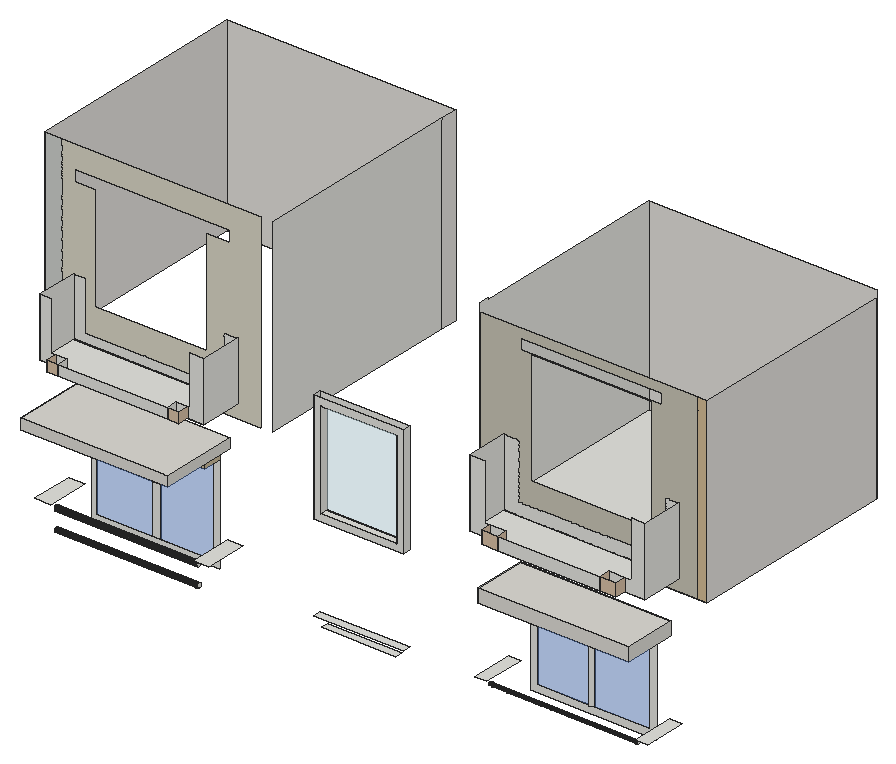
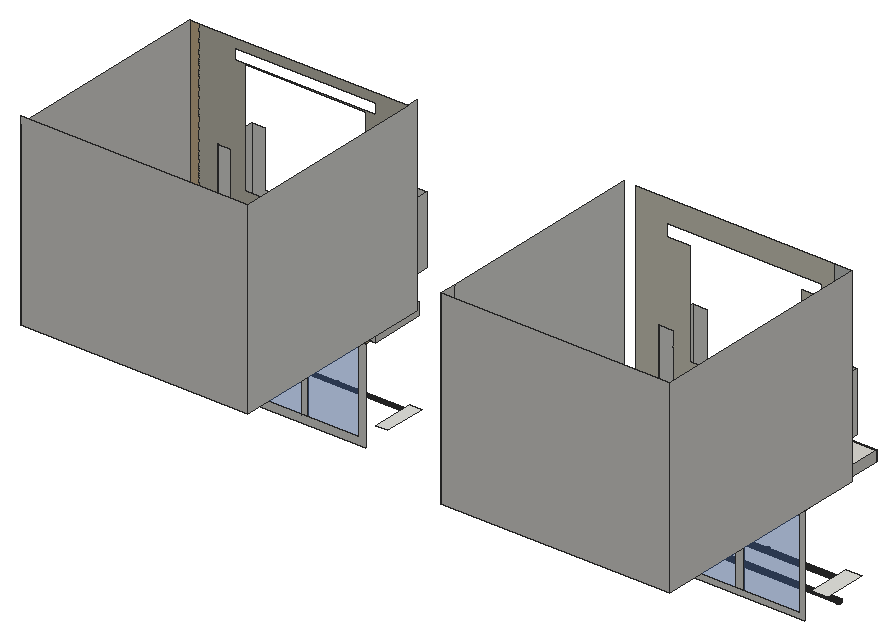
# SketchUp Ruby script. Lengths in inches.
U = 1.inch
M = Sketchup.active_model
def pt(a) = Geom::Point3d.new(a.map { |v| v * U })
def face(e, loops, mat)
  f = e.add_face(loops[0].map { |a| pt(a) })
  loops[1..].each { |l| e.add_face(l.map { |a| pt(a) }).erase! }
  f.material = f.back_material = mat if mat
  f
end
# faces: each face lists its corners as indices into pts; further lists are holes
def faces(e, pts, list, mat = nil) = list.each { |f| face(e, (f[0].is_a?(Array) ? f : [f]).map { |l| l.map { |i| pts[i] } }, mat) }
# xy, xz, yz: faces in a plane at the given z, y or x. An outline is a flat list of corners, or four numbers for a rectangle; further outlines are holes
def ring(l) = l.size == 4 ? [[l[0], l[1]], [l[2], l[1]], [l[2], l[3]], [l[0], l[3]]] : l.each_slice(2).to_a
def flat(e, list, mat, &to3) = list.each { |f| face(e, (f[0].is_a?(Array) ? f : [f]).map { |l| ring(l).map { |u, v| to3.(u, v) } }, mat) }
def xy(e, z, list, mat = nil) = flat(e, list, mat) { |x, y| [x, y, z] }
def xz(e, y, list, mat = nil) = flat(e, list, mat) { |x, z| [x, y, z] }
def yz(e, x, list, mat = nil) = flat(e, list, mat) { |y, z| [x, y, z] }
def lines(e, pts, list) = list.each { |a, b| e.add_line(pt(pts[a]), pt(pts[b])) }
# prism: a flat outline (further loops are holes) pulled along v
def prism(e, loops, v, mat = nil)
  f = face(e, loops, mat); d = Geom::Vector3d.new(v.map { |x| x * U })
  f.pushpull(f.normal.samedirection?(d) ? d.length : -d.length)
end
def box(e, o, s, mat = nil) = prism(e, [[o, [o[0] + s[0], o[1], o[2]], [o[0] + s[0], o[1] + s[1], o[2]], [o[0], o[1] + s[1], o[2]]]], [0, 0, s[2]], mat)
def at(x, y, z, deg = 0) = Geom::Transformation.translation(pt([x, y, z])) * Geom::Transformation.rotation(ORIGIN, Z_AXIS, deg.degrees)
def axes(o, x, y, z) = Geom::Transformation.new([*x, 0, *y, 0, *z, 0, *pt(o).to_a, 1])
def part(name) = M.definitions.add(name)
# library, detail: a bought-in or finely detailed component or shape, given as its bounding box
def library(name, o, s) = part(name).tap { |d| box(d.entities, o, s) }
def detail(e, o, s) = box(e.add_group.entities, o, s)
def put(e, d, t, mat = nil) = e.add_instance(d, t).tap { |i| i.material = mat if mat }
def group(e, t, mat = nil) = e.add_group.tap { |g| g.transformation = t; g.material = mat if mat }.entities
root = M.entities
M.materials.add("[Basic Tile]").color = [203, 206, 202]
M.materials.add("[Color M07]").color = [58, 58, 58]
M.materials.add("[Formica Beige]").color = [211, 187, 149]
M.materials.add("[Formica Graystone]").color = [198, 194, 180]
M.materials.add("[Formica Graystone]1").color = [216, 212, 196]
M.materials.add("[Formica Laminate Dark]").color = [50, 53, 60]
M.materials.add("[Formica Laminate Light]").color = [213, 189, 164]
M.materials.add("[Quartz Light Brown]").color = [199, 184, 152]
M.materials.add("[Terrazzo Tile Accent]").color = [224, 221, 217]
M.materials.add("[Terrazzo Tile Light]").color = [219, 217, 210]
M.materials.add("[Translucent Glass Blue]").color = [85, 126, 201]
M.materials["[Translucent Glass Blue]"].alpha = 0.5
M.materials.add("[Translucent Glass Safety]").color = [204, 235, 244]
M.materials["[Translucent Glass Safety]"].alpha = 0.5
xy(root,378.64,[[183.77,109.54,226.43,114.1]])
xy(root,383,[[179.41,109.54,230.79,114.1]])
xy(root,395.85,[[296.64,90.87,296.85,90.9,297.04,90.98,297.21,91.11,297.34,91.28,297.42,91.47,297.45,91.68,297.42,91.89,297.34,92.09,297.21,92.26,297.04,92.39,296.85,92.47,296.64,92.5,296.43,92.47,296.23,92.39,296.0625,92.26,295.93,92.09,295.85,91.89,295.82,91.68,295.85,91.47,295.93,91.28,296.0625,91.11,296.23,90.98,296.43,90.9]],"[Formica Laminate Dark]")
xy(root,395.97,[[324.82,90.87,325.03,90.9,325.23,90.98,325.4,91.11,325.53,91.28,325.61,91.47,325.64,91.68,325.61,91.89,325.53,92.09,325.4,92.26,325.23,92.39,325.03,92.47,324.82,92.5,324.61,92.47,324.42,92.39,324.25,92.26,324.12,92.09,324.04,91.89,324.01,91.68,324.04,91.47,324.12,91.28,324.25,91.11,324.42,90.98,324.61,90.9]],"[Formica Laminate Dark]")
xy(root,396.04,[[305.39,90.87,305.6,90.9,305.79,90.98,305.96,91.11,306.09,91.28,306.17,91.47,306.2,91.68,306.17,91.89,306.09,92.09,305.96,92.26,305.79,92.39,305.6,92.47,305.39,92.5,305.18,92.47,304.98,92.39,304.8125,92.26,304.68,92.09,304.6,91.89,304.57,91.68,304.6,91.47,304.68,91.28,304.8125,91.11,304.98,90.98,305.18,90.9],[330.07,90.87,330.28,90.9,330.48,90.98,330.65,91.11,330.78,91.28,330.86,91.47,330.89,91.68,330.86,91.89,330.78,92.09,330.65,92.26,330.48,92.39,330.28,92.47,330.07,92.5,329.86,92.47,329.67,92.39,329.5,92.26,329.37,92.09,329.29,91.89,329.26,91.68,329.29,91.47,329.37,91.28,329.5,91.11,329.67,90.98,329.86,90.9]],"[Formica Laminate Dark]")
xy(root,396.16,[[310.2,90.87,310.41,90.9,310.6,90.98,310.77,91.11,310.9,91.28,310.98,91.47,311.01,91.68,310.98,91.89,310.9,92.09,310.77,92.26,310.6,92.39,310.41,92.47,310.2,92.5,309.99,92.47,309.79,92.39,309.625,92.26,309.49,92.09,309.41,91.89,309.39,91.68,309.41,91.47,309.49,91.28,309.625,91.11,309.79,90.98,309.99,90.9],[340.51,90.87,340.72,90.9,340.92,90.98,341.09,91.11,341.21,91.28,341.3,91.47,341.32,91.68,341.3,91.89,341.21,92.09,341.09,92.26,340.92,92.39,340.72,92.47,340.51,92.5,340.3,92.47,340.1,92.39,339.9375,92.26,339.81,92.09,339.73,91.89,339.7,91.68,339.73,91.47,339.81,91.28,339.9375,91.11,340.1,90.98,340.3,90.9],[345.89,90.87,346.1,90.9,346.29,90.98,346.46,91.11,346.59,91.28,346.67,91.47,346.7,91.68,346.67,91.89,346.59,92.09,346.46,92.26,346.29,92.39,346.1,92.47,345.89,92.5,345.68,92.47,345.48,92.39,345.3125,92.26,345.18,92.09,345.1,91.89,345.07,91.68,345.1,91.47,345.18,91.28,345.3125,91.11,345.48,90.98,345.68,90.9]],"[Formica Laminate Dark]")
xy(root,396.29,[[319.89,90.87,320.1,90.9,320.29,90.98,320.46,91.11,320.59,91.28,320.67,91.47,320.7,91.68,320.67,91.89,320.59,92.09,320.46,92.26,320.29,92.39,320.1,92.47,319.89,92.5,319.68,92.47,319.48,92.39,319.3125,92.26,319.18,92.09,319.1,91.89,319.07,91.68,319.1,91.47,319.18,91.28,319.3125,91.11,319.48,90.98,319.68,90.9],[356.89,90.87,357.1,90.9,357.29,90.98,357.46,91.11,357.59,91.28,357.67,91.47,357.7,91.68,357.67,91.89,357.59,92.09,357.46,92.26,357.29,92.39,357.1,92.47,356.89,92.5,356.68,92.47,356.48,92.39,356.3125,92.26,356.18,92.09,356.1,91.89,356.07,91.68,356.1,91.47,356.18,91.28,356.3125,91.11,356.48,90.98,356.68,90.9],[369.07,90.87,369.28,90.9,369.48,90.98,369.65,91.11,369.78,91.28,369.86,91.47,369.89,91.68,369.86,91.89,369.78,92.09,369.65,92.26,369.48,92.39,369.28,92.47,369.07,92.5,368.86,92.47,368.67,92.39,368.5,92.26,368.37,92.09,368.29,91.89,368.26,91.68,368.29,91.47,368.37,91.28,368.5,91.11,368.67,90.98,368.86,90.9]],"[Formica Laminate Dark]")
xy(root,396.35,[[314.77,91,315.63,91,315.77,91.11,315.9,91.28,315.98,91.47,316.01,91.68,315.98,91.89,315.9,92.09,315.77,92.26,315.6,92.39,315.41,92.47,315.2,92.5,314.99,92.47,314.79,92.39,314.625,92.26,314.49,92.09,314.41,91.89,314.39,91.68,314.41,91.47,314.49,91.28,314.625,91.11]])
xy(root,396.35,[[315.2,90.87,315.41,90.9,315.6,90.98,315.63,91,314.77,91,314.79,90.98,314.99,90.9],[351.2,90.87,351.41,90.9,351.6,90.98,351.77,91.11,351.9,91.28,351.98,91.47,352.01,91.68,351.98,91.89,351.9,92.09,351.77,92.26,351.6,92.39,351.41,92.47,351.2,92.5,350.99,92.47,350.79,92.39,350.625,92.26,350.49,92.09,350.41,91.89,350.39,91.68,350.41,91.47,350.49,91.28,350.625,91.11,350.79,90.98,350.99,90.9]],"[Formica Laminate Dark]")
xy(root,396.41,[[374.64,90.87,374.85,90.9,375.04,90.98,375.21,91.11,375.34,91.28,375.42,91.47,375.45,91.68,375.42,91.89,375.34,92.09,375.21,92.26,375.04,92.39,374.85,92.47,374.64,92.5,374.43,92.47,374.23,92.39,374.0625,92.26,373.93,92.09,373.85,91.89,373.82,91.68,373.85,91.47,373.93,91.28,374.0625,91.11,374.23,90.98,374.43,90.9]],"[Formica Laminate Dark]")
xy(root,396.54,[[363.01,90.87,363.22,90.9,363.42,90.98,363.59,91.11,363.71,91.28,363.8,91.47,363.82,91.68,363.8,91.89,363.71,92.09,363.59,92.26,363.42,92.39,363.22,92.47,363.01,92.5,362.8,92.47,362.6,92.39,362.4375,92.26,362.31,92.09,362.23,91.89,362.2,91.68,362.23,91.47,362.31,91.28,362.4375,91.11,362.6,90.98,362.8,90.9]],"[Formica Laminate Dark]")
xy(root,396.5625,[[300.61,91.03,301.54,91.03,301.65,91.11,301.78,91.28,301.86,91.47,301.89,91.68,301.86,91.89,301.78,92.09,301.65,92.26,301.48,92.39,301.28,92.47,301.07,92.5,300.86,92.47,300.67,92.39,300.5,92.26,300.37,92.09,300.29,91.89,300.26,91.68,300.29,91.47,300.37,91.28,300.5,91.11],[334.45,91.03,336.43,91.03,336.47,91.08,336.59,91.37,336.63,91.67,336.59,91.98,336.47,92.27,336.28,92.51,336.17,92.6,334.71,92.6,334.6,92.51,334.41,92.27,334.29,91.98,334.25,91.67,334.29,91.37,334.41,91.08]])
xy(root,396.5625,[[335.44,90.49,335.75,90.53,336.03,90.64,336.28,90.83,336.43,91.03,334.45,91.03,334.6,90.83,334.85,90.64,335.13,90.53],[301.07,90.87,301.28,90.9,301.48,90.98,301.54,91.03,300.61,91.03,300.67,90.98,300.86,90.9],[334.71,92.6,336.17,92.6,336.03,92.7,335.75,92.82,335.44,92.86,335.13,92.82,334.85,92.7]],"[Formica Laminate Dark]")
xy(root,397.9,[[52.52,92.0625,52.78,92.1,53.02,92.2,53.23,92.35,53.39,92.5625,53.49,92.8,53.52,93.0625,53.49,93.32,53.39,93.5625,53.23,93.77,53.02,93.93,52.78,94.03,52.52,94.0625,52.27,94.03,52.02,93.93,51.82,93.77,51.66,93.5625,51.56,93.32,51.52,93.0625,51.56,92.8,51.66,92.5625,51.82,92.35,52.02,92.2,52.27,92.1]])
xy(root,397.9,[[63.21,92.0625,63.47,92.1,63.71,92.2,63.92,92.35,64.08,92.5625,64.18,92.8,64.21,93.0625,64.18,93.32,64.08,93.5625,63.92,93.77,63.71,93.93,63.47,94.03,63.21,94.0625,62.95,94.03,62.71,93.93,62.5,93.77,62.35,93.5625,62.25,93.32,62.21,93.0625,62.25,92.8,62.35,92.5625,62.5,92.35,62.71,92.2,62.95,92.1]],"[Color M07]")
xy(root,398.08,[[47.34,92.0625,47.6,92.1,47.84,92.2,48.04,92.35,48.2,92.5625,48.3,92.8,48.34,93.0625,48.3,93.32,48.2,93.5625,48.04,93.77,47.84,93.93,47.6,94.03,47.34,94.0625,47.08,94.03,46.84,93.93,46.63,93.77,46.47,93.5625,46.37,93.32,46.34,93.0625,46.37,92.8,46.47,92.5625,46.63,92.35,46.84,92.2,47.08,92.1]])
xy(root,398.08,[[81.59,92.0625,81.85,92.1,82.09,92.2,82.29,92.35,82.45,92.5625,82.55,92.8,82.59,93.0625,82.55,93.32,82.45,93.5625,82.29,93.77,82.09,93.93,81.85,94.03,81.59,94.0625,81.33,94.03,81.09,93.93,80.88,93.77,80.72,93.5625,80.62,93.32,80.59,93.0625,80.62,92.8,80.72,92.5625,80.88,92.35,81.09,92.2,81.33,92.1]],"[Color M07]")
xy(root,398.15,[[56.96,92.0625,57.22,92.1,57.46,92.2,57.67,92.35,57.83,92.5625,57.93,92.8,57.96,93.0625,57.93,93.32,57.83,93.5625,57.67,93.77,57.46,93.93,57.22,94.03,56.96,94.0625,56.7,94.03,56.46,93.93,56.25,93.77,56.1,93.5625,56,93.32,55.96,93.0625,56,92.8,56.1,92.5625,56.25,92.35,56.46,92.2,56.7,92.1]])
xy(root,398.15,[[69.96,92.0625,70.22,92.1,70.46,92.2,70.67,92.35,70.83,92.5625,70.93,92.8,70.96,93.0625,70.93,93.32,70.83,93.5625,70.67,93.77,70.46,93.93,70.22,94.03,69.96,94.0625,69.7,94.03,69.46,93.93,69.25,93.77,69.1,93.5625,69,93.32,68.96,93.0625,69,92.8,69.1,92.5625,69.25,92.35,69.46,92.2,69.7,92.1],[76.09,92.0625,76.35,92.1,76.59,92.2,76.79,92.35,76.95,92.5625,77.05,92.8,77.09,93.0625,77.05,93.32,76.95,93.5625,76.79,93.77,76.59,93.93,76.35,94.03,76.09,94.0625,75.83,94.03,75.59,93.93,75.38,93.77,75.22,93.5625,75.12,93.32,75.09,93.0625,75.12,92.8,75.22,92.5625,75.38,92.35,75.59,92.2,75.83,92.1],[94.65,92.0625,94.91,92.1,95.15,92.2,95.36,92.35,95.52,92.5625,95.62,92.8,95.65,93.0625,95.62,93.32,95.52,93.5625,95.36,93.77,95.15,93.93,94.91,94.03,94.65,94.0625,94.39,94.03,94.15,93.93,93.94,93.77,93.78,93.5625,93.68,93.32,93.65,93.0625,93.68,92.8,93.78,92.5625,93.94,92.35,94.15,92.2,94.39,92.1]],"[Color M07]")
xy(root,398.4,[[122.21,92.0625,122.47,92.1,122.71,92.2,122.92,92.35,123.08,92.5625,123.18,92.8,123.21,93.0625,123.18,93.32,123.08,93.5625,122.92,93.77,122.71,93.93,122.47,94.03,122.21,94.0625,121.95,94.03,121.71,93.93,121.5,93.77,121.35,93.5625,121.25,93.32,121.21,93.0625,121.25,92.8,121.35,92.5625,121.5,92.35,121.71,92.2,121.95,92.1]],"[Color M07]")
xy(root,398.46,[[100.02,92.0625,100.28,92.1,100.52,92.2,100.73,92.35,100.89,92.5625,100.99,92.8,101.02,93.0625,100.99,93.32,100.89,93.5625,100.73,93.77,100.52,93.93,100.28,94.03,100.02,94.0625,99.77,94.03,99.52,93.93,99.32,93.77,99.16,93.5625,99.06,93.32,99.02,93.0625,99.06,92.8,99.16,92.5625,99.32,92.35,99.52,92.2,99.77,92.1]],"[Color M07]")
xy(root,398.47,[[287.58,89.73,294.32,114.1],[379.76,89.73,386.54,114.1]])
xy(root,398.52,[[105.1,92.28,106.32,92.28,106.42,92.35,106.58,92.5625,106.68,92.8,106.71,93.0625,106.68,93.32,106.58,93.5625,106.42,93.77,106.21,93.93,105.97,94.03,105.71,94.0625,105.45,94.03,105.21,93.93,105,93.77,104.85,93.5625,104.75,93.32,104.71,93.0625,104.75,92.8,104.85,92.5625,105,92.35],[111.17,92.28,112.38,92.28,112.48,92.35,112.64,92.5625,112.74,92.8,112.77,93.0625,112.74,93.32,112.64,93.5625,112.48,93.77,112.27,93.93,112.03,94.03,111.77,94.0625,111.52,94.03,111.27,93.93,111.07,93.77,110.91,93.5625,110.81,93.32,110.77,93.0625,110.81,92.8,110.91,92.5625,111.07,92.35]])
xy(root,398.52,[[105.71,92.0625,105.97,92.1,106.21,92.2,106.32,92.28,105.1,92.28,105.21,92.2,105.45,92.1],[111.77,92.0625,112.03,92.1,112.27,92.2,112.38,92.28,111.17,92.28,111.27,92.2,111.52,92.1]],"[Color M07]")
xy(root,398.65,[[117.4,92.0625,117.66,92.1,117.9,92.2,118.11,92.35,118.27,92.5625,118.37,92.8,118.4,93.0625,118.37,93.32,118.27,93.5625,118.11,93.77,117.9,93.93,117.66,94.03,117.4,94.0625,117.14,94.03,116.9,93.93,116.69,93.77,116.53,93.5625,116.43,93.32,116.4,93.0625,116.43,92.8,116.53,92.5625,116.69,92.35,116.9,92.2,117.14,92.1]],"[Color M07]")
xy(root,398.83,[[86.3,92.4,89.26,92.4,89.35,92.62,89.41,93.04,89.35,93.46,89.1875,93.85,88.93,94.19,88.59,94.45,88.31,94.57,87.26,94.57,86.97,94.45,86.63,94.19,86.375,93.85,86.21,93.46,86.16,93.04,86.21,92.62],[87.26,94.57,88.31,94.57,88.2,94.61,87.78,94.67,87.36,94.61]])
xy(root,398.83,[[87.78,91.42,88.2,91.47,88.59,91.63,88.93,91.89,89.1875,92.23,89.26,92.4,86.3,92.4,86.375,92.23,86.63,91.89,86.97,91.63,87.36,91.47]],"[Color M07]")
xy(root,401.52,[[35.74,89.73,44.74,114.1],[126.56,89.73,135.17,114.1]])
xy(root,432.625,[[179.41,109.54,230.79,114.1]])
xy(root,436.61,[[183.4,109.54,226.8,114.1]])
xy(root,438.74,[[299.92,104.54,372.17,114.1]],"[Quartz Light Brown]")
xy(root,439.98,[[299.92,104.54,372.17,105.1],[299.92,105.1,372.17,114.1]])
xy(root,440.81,[[48.8,103.54,121.8,114.1]],"[Quartz Light Brown]")
xy(root,441.22,[[299.92,105.1,372.17,114.1]])
xy(root,441.22,[[[294.2,83.54,294.2,114.1,299.92,114.1,299.92,105.1,372.17,105.1,372.17,114.1,380.45,114.1,380.45,83.54],[373.86,85.05,374.25,85.1,374.61,85.25,374.92,85.49,375.16,85.8,375.3125,86.17,375.36,86.55,375.3125,86.94,375.16,87.3,374.92,87.61,374.61,87.85,374.25,88,373.86,88.05,373.47,88,373.11,87.85,372.8,87.61,372.5625,87.3,372.41,86.94,372.36,86.55,372.41,86.17,372.5625,85.8,372.8,85.49,373.11,85.25,373.47,85.1],[299.55,85.05,299.9375,85.1,300.3,85.25,300.61,85.49,300.85,85.8,301,86.17,301.05,86.55,301,86.94,300.85,87.3,300.61,87.61,300.3,87.85,299.9375,88,299.55,88.05,299.16,88,298.8,87.85,298.49,87.61,298.25,87.3,298.1,86.94,298.05,86.55,298.1,86.17,298.25,85.8,298.49,85.49,298.8,85.25,299.16,85.1]]],"[Terrazzo Tile Light]")
xy(root,444.62,[[48.8,103.54,121.8,107.85],[48.8,107.85,121.8,114.1]])
xy(root,448.43,[[48.8,107.85,121.8,114.1]])
xy(root,448.43,[[43.4,69.48,48.8,114.1],[[48.8,69.48,121.8,107.85],[119,85,119.42,85.06,119.8125,85.22,120.15,85.48,120.41,85.82,120.57,86.21,120.625,86.63,120.57,87.05,120.41,87.44,120.15,87.78,119.8125,88.04,119.42,88.2,119,88.25,118.58,88.2,118.1875,88.04,117.85,87.78,117.59,87.44,117.43,87.05,117.375,86.63,117.43,86.21,117.59,85.82,117.85,85.48,118.1875,85.22,118.58,85.06],[51.5,85,51.92,85.06,52.3125,85.22,52.65,85.48,52.91,85.82,53.07,86.21,53.125,86.63,53.07,87.05,52.91,87.44,52.65,87.78,52.3125,88.04,51.92,88.2,51.5,88.25,51.08,88.2,50.6875,88.04,50.35,87.78,50.09,87.44,49.93,87.05,49.875,86.63,49.93,86.21,50.09,85.82,50.35,85.48,50.6875,85.22,51.08,85.06]],[121.8,69.48,127.71,114.1]],"[Terrazzo Tile Light]")
xy(root,448.85,[[294.2,83.54,380.45,114.1]],"[Terrazzo Tile Light]")
xy(root,454.37,[[43.4,69.48,127.71,114.1]],"[Terrazzo Tile Light]")
xy(root,465.6875,[[270.97,114.1,401.16,235.11]])
xy(root,472.29,[[305.49,83.42,305.49,89.73,284.68,89.73,284.68,114.1,384.86,114.1,384.86,89.73,364.3,89.73,364.3,83.42]])
xy(root,472.29,[[296.37,83.42,305.49,89.73],[364.3,83.42,373.43,89.73]],"[Formica Laminate Light]")
xy(root,473.3,[[53.75,83.48,53.75,89.73,38.09,89.73,38.09,114.1,132.15,114.1,132.15,89.73,116.48,89.73,116.48,83.48]])
xy(root,473.3,[[47.29,83.48,53.75,89.73],[116.48,83.48,122.94,89.73]],"[Formica Laminate Light]")
xz(root,69.48,[[43.4,448.43,127.71,454.37]],"[Terrazzo Tile Light]")
xz(root,83.42,[[305.49,472.29,364.3,479.47]])
xz(root,83.42,[[296.37,472.29,305.49,479.47],[364.3,472.29,373.43,479.47]],"[Formica Laminate Light]")
xz(root,83.48,[[53.75,473.3,116.48,479.18]])
xz(root,83.48,[[47.29,473.3,53.75,479.18],[116.48,473.3,122.94,479.18]],"[Formica Laminate Light]")
xz(root,83.54,[[294.2,441.22,380.45,448.85]],"[Terrazzo Tile Light]")
xz(root,89.73,[[284.68,472.29,296.37,472.29,296.37,479.47,293.32,479.47,293.32,511.22,284.68,511.22],[296.37,472.29,305.49,479.47],[364.3,472.29,373.43,479.47],[373.43,472.29,384.86,472.29,384.86,511.22,377.32,511.22,377.32,479.47,373.43,479.47],[38.09,473.3,47.29,473.3,47.29,479.18,44.94,479.18,44.94,506.99,38.09,506.99],
  [47.29,473.3,53.75,479.18],[116.48,473.3,122.94,479.18],[122.94,473.3,132.15,473.3,132.15,506.99,124.21,506.99,124.21,479.18,122.94,479.18]])
xz(root,103.54,[[48.8,440.81,121.8,444.62]],"[Quartz Light Brown]")
xz(root,104.54,[[299.92,438.74,372.17,439.98]],"[Quartz Light Brown]")
xz(root,105.1,[[299.92,439.98,372.17,441.22]],"[Quartz Light Brown]")
xz(root,107.85,[[48.8,444.62,121.8,448.43]],"[Quartz Light Brown]")
xz(root,109.54,[[[179.41,432.625,230.79,496.3125],[183.4,436.61,226.8,492.32]]])
xz(root,114.1,[[[48.8,384.74,121.8,440.81],[51.8,387.74,118.8,437.8125]],[[299.92,385.12,372.17,438.74],[303.95,389.15,368.13,436.39]],[83.51,387.74,88.39,437.8125],[333.49,389.15,336.84,436.39],[[179.41,432.625,230.79,496.3125],[183.4,436.61,226.8,492.32]],
  [299.92,438.74,372.17,439.98],[299.92,439.98,372.17,441.22],[48.8,440.81,121.8,444.62],[294.2,441.22,380.45,448.85],[48.8,444.62,121.8,448.43],
  [43.4,448.43,127.71,454.37],[284.68,472.29,284.68,511.22,293.32,511.22,293.32,479.47,377.32,479.47,377.32,511.22,384.86,511.22,384.86,472.29],[38.09,473.3,38.09,506.99,44.94,506.99,44.94,479.18,124.21,479.18,124.21,506.99,132.15,506.99,132.15,473.3]])
xz(root,114.1,[[21.57,465.6875,31.29,573.6875]],"[Basic Tile]")
xz(root,114.1,[[395.49,465.6875,401.16,569]],"[Formica Beige]")
xz(root,114.1,[[[270.97,465.6875,395.49,569],[299.93,492.45,369.18,557.7],[284.68,472.29,284.68,511.22,293.32,511.22,293.32,479.47,377.32,479.47,377.32,511.22,384.86,511.22,384.86,472.29],[294.48,557.86,375.23,564.11]]],"[Formica Graystone]")
xz(root,114.1,[[[31.29,465.6875,145.58,573.6875],[50.46,494.26,50.46,554.07,38.67,554.07,38.67,560.89,127.48,560.89,127.48,554.07,114.59,554.07,114.59,494.26],[38.09,473.3,38.09,506.99,44.94,506.99,44.94,479.18,124.21,479.18,124.21,506.99,132.15,506.99,132.15,473.3]]],"[Formica Graystone]1")
xz(root,114.1,[[51.8,387.74,83.51,437.8125],[88.39,387.74,118.8,437.8125],[303.95,389.15,333.49,436.39],[336.84,389.15,368.13,436.39]],"[Translucent Glass Blue]")
xz(root,114.1,[[183.4,436.61,226.8,492.32]],"[Translucent Glass Safety]")
xz(root,235.11,[[270.97,465.6875,401.16,573]],"[Terrazzo Tile Accent]")
xz(root,244.83,[[21.57,465.6875,152.39,573.6875]],"[Terrazzo Tile Accent]")
yz(root,21.57,[[114.1,465.6875,244.83,573.6875]],"[Terrazzo Tile Accent]")
yz(root,38.09,[[89.73,473.3,114.1,506.99]])
yz(root,43.4,[[69.48,448.43,114.1,454.37]],"[Terrazzo Tile Light]")
yz(root,47.29,[[83.48,473.3,89.73,479.18]],"[Formica Laminate Light]")
yz(root,48.8,[[103.54,440.81,114.1,444.62],[107.85,444.62,114.1,448.43]],"[Quartz Light Brown]")
yz(root,53.75,[[83.48,473.3,89.73,479.18]])
yz(root,116.48,[[83.48,473.3,89.73,479.18]])
yz(root,121.8,[[103.54,440.81,114.1,444.62],[107.85,444.62,114.1,448.43]],"[Quartz Light Brown]")
yz(root,122.94,[[83.48,473.3,89.73,479.18]],"[Formica Laminate Light]")
yz(root,126.56,[[93.62,385.75,93.93,385.79,94.21,385.91,94.46,386.1,94.65,386.34,94.77,386.63,94.81,386.9375,94.77,387.25,94.65,387.53,94.46,387.78,94.21,387.97,93.93,388.09,93.62,388.125,93.3125,388.09,93.03,387.97,92.78,387.78,92.59,387.53,92.47,387.25,92.43,386.9375,92.47,386.63,92.59,386.34,92.78,386.1,93.03,385.91,93.3125,385.79],[93.49,396.95,93.81,396.99,94.11,397.12,94.37,397.32,94.57,397.58,94.69,397.88,94.74,398.2,94.69,398.52,94.57,398.83,94.37,399.09,94.11,399.28,93.81,399.41,93.49,399.45,93.16,399.41,92.86,399.28,92.6,399.09,92.4,398.83,92.28,398.52,92.24,398.2,92.28,397.88,92.4,397.58,92.6,397.32,92.86,397.12,93.16,396.99]])
yz(root,127.71,[[69.48,448.43,114.1,454.37]],"[Terrazzo Tile Light]")
yz(root,132.15,[[89.73,473.3,114.1,506.99]])
yz(root,152.39,[[114.1,465.6875,235.11,573.6875]])
yz(root,152.39,[[235.11,465.6875,244.83,573.6875]],"[Terrazzo Tile Accent]")
yz(root,179.41,[[109.54,432.625,114.1,496.3125]])
yz(root,183.4,[[109.54,436.61,114.1,492.32]])
yz(root,226.8,[[109.54,436.61,114.1,492.32]])
yz(root,230.79,[[109.54,432.625,114.1,496.3125]])
yz(root,270.97,[[114.1,465.6875,235.11,465.6875,235.11,573,119.66,573,119.66,573.6875,114.1,573.6875]])
yz(root,284.68,[[89.73,472.29,114.1,511.22]])
yz(root,294.2,[[83.54,441.22,114.1,448.85]],"[Terrazzo Tile Light]")
yz(root,296.37,[[83.42,472.29,89.73,479.47]],"[Formica Laminate Light]")
yz(root,299.92,[[104.54,438.74,114.1,439.98],[105.1,439.98,114.1,441.22]],"[Quartz Light Brown]")
yz(root,305.49,[[83.42,472.29,89.73,479.47]],"[Formica Laminate Light]")
yz(root,364.3,[[83.42,472.29,89.73,479.47]],"[Formica Laminate Light]")
yz(root,372.17,[[104.54,438.74,114.1,439.98],[105.1,439.98,114.1,441.22]],"[Quartz Light Brown]")
yz(root,373.43,[[83.42,472.29,89.73,479.47]],"[Formica Laminate Light]")
yz(root,379.76,[[91.8125,395.54,92.02,395.57,92.22,395.65,92.39,395.78,92.52,395.95,92.6,396.14,92.625,396.35,92.6,396.5625,92.52,396.76,92.39,396.93,92.22,397.06,92.02,397.14,91.8125,397.16,91.6,397.14,91.41,397.06,91.24,396.93,91.11,396.76,91.03,396.5625,91,396.35,91.03,396.14,91.11,395.95,91.24,395.78,91.41,395.65,91.6,395.57]])
yz(root,380.45,[[83.54,441.22,114.1,448.85]],"[Terrazzo Tile Light]")
yz(root,384.86,[[89.73,472.29,114.1,511.22]])
yz(root,401.16,[[114.1,465.6875,235.11,569]],"[Terrazzo Tile Accent]")
p = [[126.56,93.3125,385.79],[126.56,93.03,385.91],[44.74,93.03,385.91],[44.74,93.3125,385.79],[126.56,93.62,385.75],[44.74,93.62,385.75],
  [126.56,93.93,385.79],[44.74,93.93,385.79],[46.84,93.93,385.79],[47.84,93.93,385.79],[52.02,93.93,385.79],[53.02,93.93,385.79],
  [56.46,93.93,385.79],[57.46,93.93,385.79],[62.71,93.93,385.79],[63.71,93.93,385.79],[69.46,93.93,385.79],[70.46,93.93,385.79],
  [75.59,93.93,385.79],[76.59,93.93,385.79],[81.09,93.93,385.79],[82.09,93.93,385.79],[94.15,93.93,385.79],[95.15,93.93,385.79],
  [99.52,93.93,385.79],[100.52,93.93,385.79],[105.21,93.93,385.79],[106.21,93.93,385.79],[111.27,93.93,385.79],[112.27,93.93,385.79],
  [116.9,93.93,385.79],[117.9,93.93,385.79],[121.71,93.93,385.79],[122.71,93.93,385.79],[126.56,94.21,385.91],[44.74,94.21,385.91],
  [126.56,92.78,386.1],[44.74,92.78,386.1],[126.56,94.46,386.1],[44.74,94.46,386.1],[126.56,92.59,386.34],[44.74,92.59,386.34],
  [126.56,94.65,386.34],[44.74,94.65,386.34],[126.56,92.47,386.63],[44.74,92.47,386.63],[126.56,94.77,386.63],[44.74,94.77,386.63],
  [126.56,92.43,386.9375],[44.74,92.43,386.9375],[126.56,94.81,386.9375],[44.74,94.81,386.9375],[126.56,92.47,387.25],[44.74,92.47,387.25],
  [126.56,94.77,387.25],[44.74,94.77,387.25],[126.56,92.59,387.53],[44.74,92.59,387.53],[126.56,94.65,387.53],[44.74,94.65,387.53],
  [126.56,92.78,387.78],[44.74,92.78,387.78],[126.56,94.46,387.78],[44.74,94.46,387.78],[126.56,93.03,387.97],[44.74,93.03,387.97],
  [126.56,94.21,387.97],[44.74,94.21,387.97],[126.56,93.3125,388.09],[44.74,93.3125,388.09],[126.56,93.93,388.09],[44.74,93.93,388.09],
  [46.84,93.93,388.09],[47.84,93.93,388.09],[52.02,93.93,388.09],[53.02,93.93,388.09],[56.46,93.93,388.09],[57.46,93.93,388.09],
  [62.71,93.93,388.09],[63.71,93.93,388.09],[69.46,93.93,388.09],[70.46,93.93,388.09],[75.59,93.93,388.09],[76.59,93.93,388.09],
  [81.09,93.93,388.09],[82.09,93.93,388.09],[94.15,93.93,388.09],[95.15,93.93,388.09],[99.52,93.93,388.09],[100.52,93.93,388.09],
  [105.21,93.93,388.09],[106.21,93.93,388.09],[111.27,93.93,388.09],[112.27,93.93,388.09],[116.9,93.93,388.09],[117.9,93.93,388.09],
  [121.71,93.93,388.09],[122.71,93.93,388.09],[126.56,93.62,388.125],[44.74,93.62,388.125],[379.76,91.8125,395.54],[379.76,91.6,395.57],
  [294.32,91.6,395.57],[294.32,91.8125,395.54],[379.76,92.02,395.57],[294.32,92.02,395.57],[379.76,91.41,395.65],[379.76,91.24,395.78],
  [294.32,91.24,395.78],[294.32,91.41,395.65],[379.76,92.22,395.65],[294.32,92.22,395.65],[379.76,92.39,395.78],[294.32,92.39,395.78],
  [296.23,92.39,395.78],[297.04,92.39,395.78],[300.67,92.39,395.78],[301.48,92.39,395.78],[304.98,92.39,395.78],[305.79,92.39,395.78],
  [309.79,92.39,395.78],[310.6,92.39,395.78],[314.79,92.39,395.78],[315.6,92.39,395.78],[319.48,92.39,395.78],[320.29,92.39,395.78],
  [324.42,92.39,395.78],[325.23,92.39,395.78],[329.67,92.39,395.78],[330.48,92.39,395.78],[340.1,92.39,395.78],[340.92,92.39,395.78],
  [345.48,92.39,395.78],[346.29,92.39,395.78],[350.79,92.39,395.78],[351.6,92.39,395.78],[356.48,92.39,395.78],[357.29,92.39,395.78],
  [362.6,92.39,395.78],[363.42,92.39,395.78],[368.67,92.39,395.78],[369.48,92.39,395.78],[374.23,92.39,395.78],[375.04,92.39,395.78],
  [379.76,91.11,395.95],[375.21,91.11,395.95],[374.0625,91.11,395.95],[369.65,91.11,395.95],[368.5,91.11,395.95],[363.59,91.11,395.95],
  [362.4375,91.11,395.95],[357.46,91.11,395.95],[356.3125,91.11,395.95],[351.77,91.11,395.95],[350.625,91.11,395.95],[346.46,91.11,395.95],
  [345.3125,91.11,395.95],[341.09,91.11,395.95],[339.9375,91.11,395.95],[330.65,91.11,395.95],[329.5,91.11,395.95],[325.4,91.11,395.95],
  [324.25,91.11,395.95],[320.46,91.11,395.95],[319.3125,91.11,395.95],[315.77,91.11,395.95],[314.625,91.11,395.95],[310.77,91.11,395.95],
  [309.625,91.11,395.95],[305.96,91.11,395.95],[304.8125,91.11,395.95],[301.65,91.11,395.95],[300.5,91.11,395.95],[294.32,91.11,395.95],
  [379.76,92.52,395.95],[294.32,92.52,395.95],[379.76,91.03,396.14],[294.32,91.03,396.14],[379.76,92.6,396.14],[294.32,92.6,396.14],
  [379.76,91,396.35],[315.63,91,396.35],[314.77,91,396.35],[294.32,91,396.35],[379.76,92.625,396.35],[294.32,92.625,396.35],
  [379.76,91.03,396.5625],[336.43,91.03,396.5625],[334.45,91.03,396.5625],[301.54,91.03,396.5625],[300.61,91.03,396.5625],[294.32,91.03,396.5625],
  [379.76,92.6,396.5625],[294.32,92.6,396.5625],[334.71,92.6,396.5625],[336.17,92.6,396.5625],[379.76,91.11,396.76],[294.32,91.11,396.76],
  [379.76,92.52,396.76],[294.32,92.52,396.76],[379.76,91.24,396.93],[294.32,91.24,396.93],[379.76,92.39,396.93],[294.32,92.39,396.93],
  [379.76,91.41,397.06],[294.32,91.41,397.06],[379.76,92.22,397.06],[294.32,92.22,397.06],[126.56,93.16,396.99],[126.56,92.86,397.12],
  [44.74,92.86,397.12],[44.74,93.16,396.99],[126.56,93.49,396.95],[44.74,93.49,396.95],[126.56,93.81,396.99],[44.74,93.81,396.99],
  [126.56,94.11,397.12],[44.74,94.11,397.12],[379.76,91.6,397.14],[294.32,91.6,397.14],[379.76,91.8125,397.16],[294.32,91.8125,397.16],
  [379.76,92.02,397.14],[294.32,92.02,397.14],[126.56,92.6,397.32],[44.74,92.6,397.32],[126.56,94.37,397.32],[44.74,94.37,397.32],
  [126.56,92.4,397.58],[44.74,92.4,397.58],[126.56,94.57,397.58],[44.74,94.57,397.58],[126.56,92.28,397.88],[44.74,92.28,397.88],
  [126.56,94.69,397.88],[44.74,94.69,397.88],[126.56,92.24,398.2],[44.74,92.24,398.2],[126.56,94.74,398.2],[44.74,94.74,398.2],
  [126.56,92.28,398.52],[112.38,92.28,398.52],[111.17,92.28,398.52],[106.32,92.28,398.52],[105.1,92.28,398.52],[44.74,92.28,398.52],
  [126.56,94.69,398.52],[44.74,94.69,398.52],[126.56,92.4,398.83],[89.26,92.4,398.83],[86.3,92.4,398.83],[44.74,92.4,398.83],
  [126.56,94.57,398.83],[44.74,94.57,398.83],[87.26,94.57,398.83],[88.31,94.57,398.83],[126.56,92.6,399.09],[44.74,92.6,399.09],
  [126.56,94.37,399.09],[44.74,94.37,399.09],[126.56,92.86,399.28],[44.74,92.86,399.28],[126.56,94.11,399.28],[44.74,94.11,399.28],
  [126.56,93.16,399.41],[44.74,93.16,399.41],[126.56,93.81,399.41],[44.74,93.81,399.41],[126.56,93.49,399.45],[44.74,93.49,399.45]]
faces(root,p,[[0,1,2,3],[4,0,3,5],[6,4,5,7,8,9,10,11,12,13,14,15,16,17,18,19,20,21,22,23,24,25,26,27,28,29,30,31,32,33],[34,6,33,32,31,30,29,28,27,26,25,24,23,22,21,20,19,18,17,16,15,14,13,12,11,10,9,8,7,35],[1,36,37,2],[38,34,35,39],[36,40,41,37],[42,38,39,43],
  [40,44,45,41],[46,42,43,47],[44,48,49,45],[50,46,47,51],[48,52,53,49],[54,50,51,55],[52,56,57,53],[58,54,55,59],
  [56,60,61,57],[62,58,59,63],[60,64,65,61],[66,62,63,67],[64,68,69,65],[70,66,67,71,72,73,74,75,76,77,78,79,80,81,82,83,84,85,86,87,88,89,90,91,92,93,94,95,96,97],[68,98,99,69],[98,70,97,96,95,94,93,92,91,90,89,88,87,86,85,84,83,82,81,80,79,78,77,76,75,74,73,72,71,99],
  [208,209,210,211],[212,208,211,213],[214,212,213,215],[216,214,215,217],[209,224,225,210],[226,216,217,227],[224,228,229,225],[230,226,227,231],
  [228,232,233,229],[234,230,231,235],[232,236,237,233],[238,234,235,239],[236,240,241,242,243,244,245,237],[246,238,239,247],[240,248,249,250,251,245,244,243,242,241],[252,246,247,253,254,255],
  [248,256,257,251,250,249],[258,252,255,254,253,259],[256,260,261,257],[262,258,259,263],[260,264,265,261],[266,262,263,267],[264,268,269,265],[268,266,267,269]],"[Color M07]")
faces(root,p,[[100,101,102,103],[104,100,103,105],[106,107,108,109],[101,106,109,102],[110,104,105,111],[112,110,111,113,114,115,116,117,118,119,120,121,122,123,124,125,126,127,128,129,130,131,132,133,134,135,136,137,138,139,140,141,142,143],[107,144,145,146,147,148,149,150,151,152,153,154,155,156,157,158,159,160,161,162,163,164,165,166,167,168,169,170,171,172,173,108],[174,112,143,142,141,140,139,138,137,136,135,134,133,132,131,130,129,128,127,126,125,124,123,122,121,120,119,118,117,116,115,114,113,175],
  [144,176,177,173,172,171,170,169,168,167,166,165,164,163,162,161,160,159,158,157,156,155,154,153,152,151,150,149,148,147,146,145],[178,174,175,179],[176,180,181,182,183,177],[184,178,179,185],[180,186,187,188,189,190,191,183,182,181],[192,184,185,193,194,195],[186,196,197,191,190,189,188,187],[198,192,195,194,193,199],
  [196,200,201,197],[202,198,199,203],[200,204,205,201],[206,202,203,207],[204,218,219,205],[218,220,221,219],[220,222,223,221],[222,206,207,223]],"[Formica Laminate Dark]")
